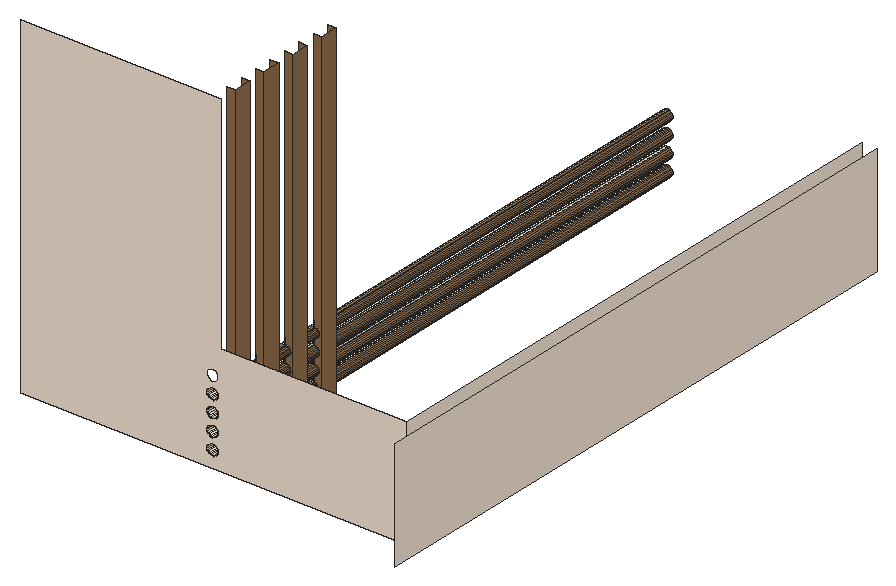
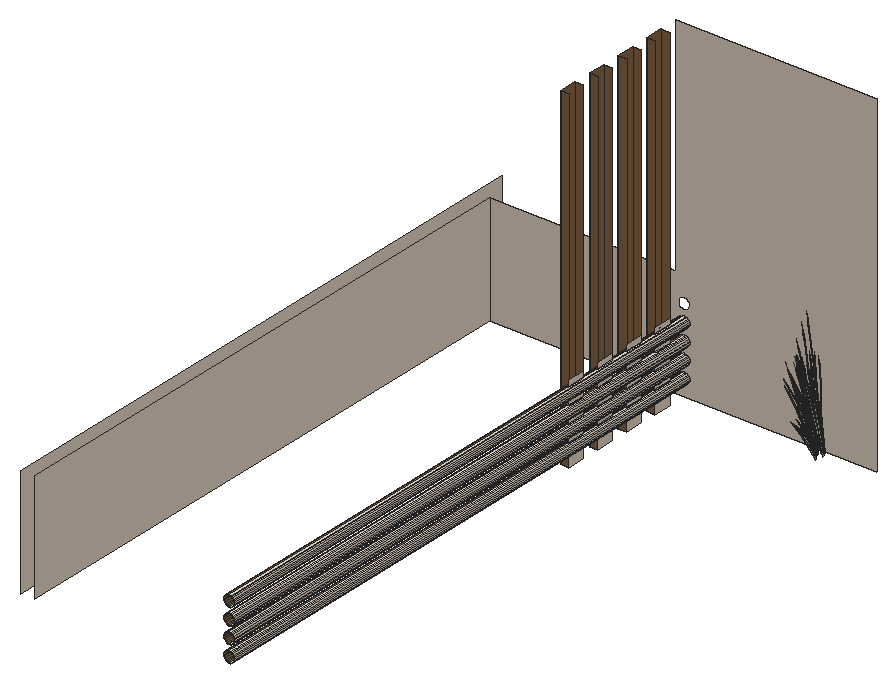
# SketchUp Ruby script. Lengths in inches.
U = 1.inch
M = Sketchup.active_model
def pt(a) = Geom::Point3d.new(a.map { |v| v * U })
def face(e, loops, mat)
  f = e.add_face(loops[0].map { |a| pt(a) })
  loops[1..].each { |l| e.add_face(l.map { |a| pt(a) }).erase! }
  f.material = f.back_material = mat if mat
  f
end
# faces: each face lists its corners as indices into pts; further lists are holes
def faces(e, pts, list, mat = nil) = list.each { |f| face(e, (f[0].is_a?(Array) ? f : [f]).map { |l| l.map { |i| pts[i] } }, mat) }
# xy, xz, yz: faces in a plane at the given z, y or x. An outline is a flat list of corners, or four numbers for a rectangle; further outlines are holes
def ring(l) = l.size == 4 ? [[l[0], l[1]], [l[2], l[1]], [l[2], l[3]], [l[0], l[3]]] : l.each_slice(2).to_a
def flat(e, list, mat, &to3) = list.each { |f| face(e, (f[0].is_a?(Array) ? f : [f]).map { |l| ring(l).map { |u, v| to3.(u, v) } }, mat) }
def xy(e, z, list, mat = nil) = flat(e, list, mat) { |x, y| [x, y, z] }
def xz(e, y, list, mat = nil) = flat(e, list, mat) { |x, z| [x, y, z] }
def yz(e, x, list, mat = nil) = flat(e, list, mat) { |y, z| [x, y, z] }
def lines(e, pts, list) = list.each { |a, b| e.add_line(pt(pts[a]), pt(pts[b])) }
# prism: a flat outline (further loops are holes) pulled along v
def prism(e, loops, v, mat = nil)
  f = face(e, loops, mat); d = Geom::Vector3d.new(v.map { |x| x * U })
  f.pushpull(f.normal.samedirection?(d) ? d.length : -d.length)
end
def box(e, o, s, mat = nil) = prism(e, [[o, [o[0] + s[0], o[1], o[2]], [o[0] + s[0], o[1] + s[1], o[2]], [o[0], o[1] + s[1], o[2]]]], [0, 0, s[2]], mat)
def at(x, y, z, deg = 0) = Geom::Transformation.translation(pt([x, y, z])) * Geom::Transformation.rotation(ORIGIN, Z_AXIS, deg.degrees)
def axes(o, x, y, z) = Geom::Transformation.new([*x, 0, *y, 0, *z, 0, *pt(o).to_a, 1])
def part(name) = M.definitions.add(name)
# library, detail: a bought-in or finely detailed component or shape, given as its bounding box
def library(name, o, s) = part(name).tap { |d| box(d.entities, o, s) }
def detail(e, o, s) = box(e.add_group.entities, o, s)
def put(e, d, t, mat = nil) = e.add_instance(d, t).tap { |i| i.material = mat if mat }
def group(e, t, mat = nil) = e.add_group.tap { |g| g.transformation = t; g.material = mat if mat }.entities
root = M.entities
M.materials.add("C01_Vanilla_Cream").color = [244, 228, 212]
M.materials.add("LightPink_Translucent").color = [144, 107, 117]
M.materials["LightPink_Translucent"].alpha = 0.75
M.materials.add("Wood_Floor_01_1K").color = [146, 111, 76]
c1 = part("blade")
p = [[2.15,0.21,22],[0,0.17,0],[0.09,0.45,0],[2.18,0.31,22],[2.29,0.31,22],[0.38,0.45,0],
  [2.48,0.24,33],[2.49,0.24,33],[2.48,0.22,33]]
faces(c1.entities,p,[[0,1,2,3],[4,5,2,3],[6,3,4,7],[8,0,3,6]])
c2 = part("seeds")
p = [[0.3,-0.1,1.38],[-0.01,-0.03,1.59],[-0.01,-0.03,0.03],[0.14,-0.07,-0.07],[0.29,-0.03,3],[0.15,0.01,3.11]]
faces(c2.entities,p,[[0,1,2,3],[1,0,4,5]],"LightPink_Translucent")
c3 = part("blade with seeds")
put(c3.entities,c1,at(0,0,0))
put(c3.entities,c2,axes([2.4,0.25,30.99],[1.5799,-0.05474,1.17369],[-0.12525,1.92788,0.29478],[-0.07173,-0.02425,1.56792]))
xy(root,12,[[357,18.46,360,24.91],[357,31.37,360,37.83],[357,44.28,360,50.74],[357,57.2,360,63.65]],"C01_Vanilla_Cream")
xz(root,12,[[[288,12,288,132,360,132,360,51.56,426.72,51.56,426.72,12],[357,16,357.52,16.07,358,16.27,358.41,16.59,358.73,17,358.93,17.48,359,18,358.93,18.52,358.73,19,358.41,19.41,358,19.73,357.52,19.93,357,20,356.48,19.93,356,19.73,355.59,19.41,355.27,19,355.07,18.52,355,18,355.07,17.48,355.27,17,355.59,16.59,356,16.27,356.48,16.07],[357,22,357.52,22.07,358,22.27,358.41,22.59,358.73,23,358.93,23.48,359,24,358.93,24.52,358.73,25,358.41,25.41,358,25.73,357.52,25.93,357,26,356.48,25.93,356,25.73,355.59,25.41,355.27,25,355.07,24.52,355,24,355.07,23.48,355.27,23,355.59,22.59,356,22.27,356.48,22.07],[357,28,357.52,28.07,358,28.27,358.41,28.59,358.73,29,358.93,29.48,359,30,358.93,30.52,358.73,31,358.41,31.41,358,31.73,357.52,31.93,357,32,356.48,31.93,356,31.73,355.59,31.41,355.27,31,355.07,30.52,355,30,355.07,29.48,355.27,29,355.59,28.59,356,28.27,356.48,28.07],[357,40,357.52,40.07,358,40.27,358.41,40.59,358.73,41,358.93,41.48,359,42,358.93,42.52,358.73,43,358.41,43.41,358,43.73,357.52,43.93,357,44,356.48,43.93,356,43.73,355.59,43.41,355.27,43,355.07,42.52,355,42,355.07,41.48,355.27,41,355.59,40.59,356,40.27,356.48,40.07],[357,34,357.52,34.07,358,34.27,358.41,34.59,358.73,35,358.93,35.48,359,36,358.93,36.52,358.73,37,358.41,37.41,358,37.73,357.52,37.93,357,38,356.48,37.93,356,37.73,355.59,37.41,355.27,37,355.07,36.52,355,36,355.07,35.48,355.27,35,355.59,34.59,356,34.27,356.48,34.07]]],"C01_Vanilla_Cream")
xz(root,18.46,[[357,12,360,132]],"Wood_Floor_01_1K")
xz(root,24.91,[[357,12,360,132]],"Wood_Floor_01_1K")
xz(root,31.37,[[357,12,360,132]],"Wood_Floor_01_1K")
xz(root,37.83,[[357,12,360,132]],"Wood_Floor_01_1K")
xz(root,44.28,[[357,12,360,132]],"Wood_Floor_01_1K")
xz(root,50.74,[[357,12,360,132]],"Wood_Floor_01_1K")
xz(root,57.2,[[357,12,360,132]],"Wood_Floor_01_1K")
xz(root,63.65,[[357,12,360,132]],"Wood_Floor_01_1K")
yz(root,357,[[18.46,12,24.91,16],[31.37,12,37.83,16],[44.28,12,50.74,16],[57.2,12,63.65,16],[18.46,16,24.91,20],
  [31.37,16,37.83,20],[44.28,16,50.74,20],[57.2,16,63.65,20],[18.46,20,24.91,22],[31.37,20,37.83,22],
  [44.28,20,50.74,22],[57.2,20,63.65,22],[18.46,22,24.91,26],[31.37,22,37.83,26],[44.28,22,50.74,26],
  [57.2,22,63.65,26],[18.46,26,24.91,28],[31.37,26,37.83,28],[44.28,26,50.74,28],[57.2,26,63.65,28],
  [18.46,28,24.91,32],[31.37,28,37.83,32],[44.28,28,50.74,32],[57.2,28,63.65,32],[18.46,32,24.91,34],
  [31.37,32,37.83,34],[44.28,32,50.74,34],[57.2,32,63.65,34],[18.46,34,24.91,38],[31.37,34,37.83,38],
  [44.28,34,50.74,38],[57.2,34,63.65,38],[18.46,38,24.91,40],[31.37,38,37.83,40],[44.28,38,50.74,40],
  [57.2,38,63.65,40]],"C01_Vanilla_Cream")
yz(root,360,[[18.46,12,24.91,132],[31.37,12,37.83,132],[44.28,12,50.74,132],[57.2,12,63.65,132]],"Wood_Floor_01_1K")
yz(root,426.72,[[12,12,216,51.56]],"C01_Vanilla_Cream")
yz(root,432,[[0,12,216,51.56]],"C01_Vanilla_Cream")
p = [[356.48,216,16.07],[357,216,16],[357,63.65,16],[357,57.2,16],[357,50.74,16],[357,44.28,16],
  [357,37.83,16],[357,31.37,16],[357,24.91,16],[357,18.46,16],[357,12,16],[356.48,12,16.07],
  [357.52,216,16.07],[357.52,12,16.07],[356,216,16.27],[356,12,16.27],[358,216,16.27],[358,12,16.27],
  [355.59,216,16.59],[355.59,12,16.59],[358.41,216,16.59],[358.41,12,16.59],[355.27,216,17],[355.27,12,17],
  [358.73,216,17],[358.73,12,17],[355.07,216,17.48],[355.07,12,17.48],[358.93,216,17.48],[358.93,12,17.48],
  [355,216,18],[355,12,18],[359,216,18],[359,12,18],[355.07,216,18.52],[355.07,12,18.52],
  [358.93,216,18.52],[358.93,12,18.52],[355.27,216,19],[355.27,12,19],[358.73,216,19],[358.73,12,19],
  [355.59,216,19.41],[355.59,12,19.41],[358.41,216,19.41],[358.41,12,19.41],[356,216,19.73],[356,12,19.73],
  [358,216,19.73],[358,12,19.73],[356.48,216,19.93],[356.48,12,19.93],[357.52,216,19.93],[357.52,12,19.93],
  [357,216,20],[357,12,20],[357,18.46,20],[357,24.91,20],[357,31.37,20],[357,37.83,20],
  [357,44.28,20],[357,50.74,20],[357,57.2,20],[357,63.65,20],[356.48,216,22.07],[357,216,22],
  [357,63.65,22],[357,57.2,22],[357,50.74,22],[357,44.28,22],[357,37.83,22],[357,31.37,22],
  [357,24.91,22],[357,18.46,22],[357,12,22],[356.48,12,22.07],[357.52,216,22.07],[357.52,12,22.07],
  [356,216,22.27],[356,12,22.27],[358,216,22.27],[358,12,22.27],[355.59,216,22.59],[355.59,12,22.59],
  [358.41,216,22.59],[358.41,12,22.59],[355.27,216,23],[355.27,12,23],[358.73,216,23],[358.73,12,23],
  [355.07,216,23.48],[355.07,12,23.48],[358.93,216,23.48],[358.93,12,23.48],[355,216,24],[355,12,24],
  [359,216,24],[359,12,24],[355.07,216,24.52],[355.07,12,24.52],[358.93,216,24.52],[358.93,12,24.52],
  [355.27,216,25],[355.27,12,25],[358.73,216,25],[358.73,12,25],[355.59,216,25.41],[355.59,12,25.41],
  [358.41,216,25.41],[358.41,12,25.41],[356,216,25.73],[356,12,25.73],[358,216,25.73],[358,12,25.73],
  [356.48,216,25.93],[356.48,12,25.93],[357.52,216,25.93],[357.52,12,25.93],[357,216,26],[357,12,26],
  [357,18.46,26],[357,24.91,26],[357,31.37,26],[357,37.83,26],[357,44.28,26],[357,50.74,26],
  [357,57.2,26],[357,63.65,26],[356.48,216,28.07],[357,216,28],[357,63.65,28],[357,57.2,28],
  [357,50.74,28],[357,44.28,28],[357,37.83,28],[357,31.37,28],[357,24.91,28],[357,18.46,28],
  [357,12,28],[356.48,12,28.07],[357.52,216,28.07],[357.52,12,28.07],[356,216,28.27],[356,12,28.27],
  [358,216,28.27],[358,12,28.27],[355.59,216,28.59],[355.59,12,28.59],[358.41,216,28.59],[358.41,12,28.59],
  [355.27,216,29],[355.27,12,29],[358.73,216,29],[358.73,12,29],[355.07,216,29.48],[355.07,12,29.48],
  [358.93,216,29.48],[358.93,12,29.48],[355,216,30],[355,12,30],[359,216,30],[359,12,30],
  [355.07,216,30.52],[355.07,12,30.52],[358.93,216,30.52],[358.93,12,30.52],[355.27,216,31],[355.27,12,31],
  [358.73,216,31],[358.73,12,31],[355.59,216,31.41],[355.59,12,31.41],[358.41,216,31.41],[358.41,12,31.41],
  [356,216,31.73],[356,12,31.73],[358,216,31.73],[358,12,31.73],[356.48,216,31.93],[356.48,12,31.93],
  [357.52,216,31.93],[357.52,12,31.93],[357,216,32],[357,12,32],[357,18.46,32],[357,24.91,32],
  [357,31.37,32],[357,37.83,32],[357,44.28,32],[357,50.74,32],[357,57.2,32],[357,63.65,32],
  [356.48,216,34.07],[357,216,34],[357,63.65,34],[357,57.2,34],[357,50.74,34],[357,44.28,34],
  [357,37.83,34],[357,31.37,34],[357,24.91,34],[357,18.46,34],[357,12,34],[356.48,12,34.07],
  [357.52,216,34.07],[357.52,12,34.07],[356,216,34.27],[356,12,34.27],[358,216,34.27],[358,12,34.27],
  [355.59,216,34.59],[355.59,12,34.59],[358.41,216,34.59],[358.41,12,34.59],[355.27,216,35],[355.27,12,35],
  [358.73,216,35],[358.73,12,35],[355.07,216,35.48],[355.07,12,35.48],[358.93,216,35.48],[358.93,12,35.48],
  [355,216,36],[355,12,36],[359,216,36],[359,12,36],[355.07,216,36.52],[355.07,12,36.52],
  [358.93,216,36.52],[358.93,12,36.52],[355.27,216,37],[355.27,12,37],[358.73,216,37],[358.73,12,37],
  [355.59,216,37.41],[355.59,12,37.41],[358.41,216,37.41],[358.41,12,37.41],[356,216,37.73],[356,12,37.73],
  [358,216,37.73],[358,12,37.73],[357,216,38],[356.48,216,37.93],[356.48,12,37.93],[357,12,38],
  [357,18.46,38],[357,24.91,38],[357,31.37,38],[357,37.83,38],[357,44.28,38],[357,50.74,38],
  [357,57.2,38],[357,63.65,38],[357.52,216,37.93],[357.52,12,37.93]]
faces(root,p,[[0,1,2,3,4,5,6,7,8,9,10,11],[14,0,11,15],[18,14,15,19],[22,18,19,23],[26,22,23,27],[30,26,27,31],[34,30,31,35],[38,34,35,39],
  [42,38,39,43],[46,42,43,47],[50,46,47,51],[54,50,51,55,56,57,58,59,60,61,62,63],[64,65,66,67,68,69,70,71,72,73,74,75],[78,64,75,79],[82,78,79,83],[86,82,83,87],
  [90,86,87,91],[94,90,91,95],[98,94,95,99],[102,98,99,103],[106,102,103,107],[110,106,107,111],[114,110,111,115],[118,114,115,119,120,121,122,123,124,125,126,127],
  [128,129,130,131,132,133,134,135,136,137,138,139],[142,128,139,143],[146,142,143,147],[150,146,147,151],[154,150,151,155],[158,154,155,159],[162,158,159,163],[166,162,163,167],
  [170,166,167,171],[174,170,171,175],[178,174,175,179],[182,178,179,183,184,185,186,187,188,189,190,191],[192,193,194,195,196,197,198,199,200,201,202,203],[206,192,203,207],[210,206,207,211],[214,210,211,215],
  [218,214,215,219],[222,218,219,223],[226,222,223,227],[230,226,227,231],[234,230,231,235],[238,234,235,239],[242,243,244,245,246,247,248,249,250,251,252,253]],"C01_Vanilla_Cream")
faces(root,p,[[1,12,13,10,9,8,7,6,5,4,3,2],[12,16,17,13],[16,20,21,17],[20,24,25,21],[24,28,29,25],[28,32,33,29],[32,36,37,33],[36,40,41,37],
  [40,44,45,41],[44,48,49,45],[48,52,53,49],[52,54,63,62,61,60,59,58,57,56,55,53],[65,76,77,74,73,72,71,70,69,68,67,66],[76,80,81,77],[80,84,85,81],[84,88,89,85],
  [88,92,93,89],[92,96,97,93],[96,100,101,97],[100,104,105,101],[104,108,109,105],[108,112,113,109],[112,116,117,113],[116,118,127,126,125,124,123,122,121,120,119,117],
  [129,140,141,138,137,136,135,134,133,132,131,130],[140,144,145,141],[144,148,149,145],[148,152,153,149],[152,156,157,153],[156,160,161,157],[160,164,165,161],[164,168,169,165],
  [168,172,173,169],[172,176,177,173],[176,180,181,177],[180,182,191,190,189,188,187,186,185,184,183,181],[193,204,205,202,201,200,199,198,197,196,195,194],[204,208,209,205],[208,212,213,209],[212,216,217,213],
  [216,220,221,217],[220,224,225,221],[224,228,229,225],[228,232,233,229],[232,236,237,233],[236,240,241,237],[254,242,253,252,251,250,249,248,247,246,245,255]],"Wood_Floor_01_1K")
put(root,c3,axes([298.97,21.29,18.38],[0.34808,-0.49367,0],[0.58235,0.27531,-0.38706],[0.13264,0.0627,1.22783]))
put(root,c3,axes([299.56,21.08,17.72],[-0.08333,-0.03881,1.32257],[-0.21404,-0.4336,-0.20205],[0.14439,-0.11767,0.22528]))
put(root,c3,axes([299.1,24.23,20.39],[-0.31678,-0.30846,0.2656],[0.36171,-0.29199,-0.3429],[0.18378,0.04443,0.65611]))
put(root,c3,axes([299.29,21.59,18.12],[0.52105,0.24633,-0.37238],[-0.31144,0.44171,0],[0.11867,0.0561,1.18128]))
put(root,c3,axes([299.39,24.51,20.15],[-0.02803,0.37463,0.04823],[-0.42332,-0.01027,0.37966],[0.16216,0.0392,0.57892]))
put(root,c3,axes([299.26,25.09,17.72],[0.04056,-0.07113,1.32257],[0.51066,-0.20948,-0.20205],[0.15482,0.10842,0.22528]))
put(root,c3,axes([299.42,24.39,20.15],[-0.41051,0.32462,0.36002],[-0.35404,-0.34474,0.29685],[0.1926,0.05988,0.74497]))
put(root,c3,axes([299.54,22.12,20.11],[-0.14302,-0.44985,-0.38324],[0.54163,-0.07869,-0.29685],[0.15522,-0.12083,0.7333]))
put(root,c3,axes([300.49,24.44,19.55],[-0.10656,-0.41414,-0.02619],[0.50364,-0.09521,-0.11874],[0.10517,0.02626,0.39164]))
put(root,c3,axes([299.62,23.37,20.39],[-0.46269,-0.13744,0.2656],[0.13495,-0.40096,-0.3429],[0.18628,-0.03677,0.65611]))
put(root,c3,axes([298.53,22.53,18.15],[0.57914,0.08077,-0.46765],[-0.12221,0.49823,-0.12274],[0.17283,0.06037,1.03225]))
put(root,c3,axes([301,22.83,18.3],[-0.34516,-0.31503,-0.04866],[0.37803,-0.28865,-0.22062],[0.10711,-0.02032,0.72768]))
put(root,c3,axes([300.2,21.22,18.68],[-0.18544,0.25079,0.86145],[-0.15939,-0.33694,0.63294],[0.15316,-0.08443,0.18974]))
put(root,c3,axes([299.98,22.34,20.15],[0.3822,0.20719,0.04823],[-0.22252,0.29505,0.37966],[0.12254,-0.09539,0.57892]))
put(root,c3,axes([299.875,22.25,20.15],[0.13808,0.45342,0.36002],[-0.54163,0.07869,0.29685],[0.15963,-0.10664,0.74497]))
put(root,c3,axes([298.41,23.6,19.51],[-0.2068,-0.08488,1.28532],[0.42797,-0.35609,0.10393],[0.26673,0.16064,0.54946]))
put(root,c3,axes([301.0625,22.32,20.13],[-0.07272,-0.00374,1.33037],[-0.30197,-0.40092,-0.12571],[0.12127,-0.13182,0.23543]))
put(root,c3,axes([299.9375,22.17,20],[0.48462,-0.07041,-0.2656],[0.12797,0.4025,0.3429],[0.13888,-0.10811,0.65611]))
put(root,c3,axes([299.55,22.3,20.34],[0.29081,-0.38873,-0.53284],[0.5096,0.27626,0.0643],[0.17364,-0.14084,0.75375]))
put(root,c3,axes([300.04,23.49,20.15],[0.20448,0.33592,0.04823],[-0.37288,0.16442,0.37966],[0.16437,-0.03244,0.57892]))
put(root,c3,axes([299.55,24.39,20],[0.31678,0.30846,-0.2656],[-0.36171,0.29199,0.3429],[0.18378,0.04443,0.65611]))
put(root,c3,axes([299.19,24.43,20.38],[0.02981,-0.50103,-0.0912],[0.56442,0.01369,-0.50621],[0.21738,0.0348,0.76918]))
put(root,c3,axes([299.81,23.5,20.38],[-0.28012,-0.44611,-0.0912],[0.49717,-0.21923,-0.50621],[0.20951,-0.05886,0.76918]))
put(root,c3,axes([300,23.37,20.15],[-0.15729,0.44921,0.36002],[-0.51712,-0.15361,0.29685],[0.20336,-0.027,0.74497]))
put(root,c3,axes([299.68,24.125,20.14],[0.11943,-0.00833,1.31208],[0.32759,-0.38275,-0.2075],[0.21244,0.05052,0.10523]))
put(root,c3,axes([299.79,23.12,20.11],[0.15083,-0.44814,-0.38324],[0.51712,0.15361,-0.29685],[0.2082,-0.04109,0.7333]))
put(root,c3,axes([301.09,23.4,18.68],[-0.34399,0.08133,0.86145],[0.16192,-0.33614,0.63294],[0.18249,0.023,0.18974]))
put(root,c3,axes([299.97,21.94,18.55],[-0.19889,-0.01459,1.07251],[-0.20376,-0.39145,-0.23066],[0.24434,-0.11074,0.45856]))
put(root,c3,axes([300.11,23.32,20],[0.46269,0.13744,-0.2656],[-0.13495,0.40096,0.3429],[0.18628,-0.03677,0.65611]))
put(root,c3,axes([299.21,24.1875,20.34],[0.55654,0.01186,-0.53284],[-0.03738,0.49951,0.0643],[0.23578,0.05271,0.75375]))
put(root,c3,axes([300.34,23.24,18.09],[-0.35858,0.05912,1.06187],[-0.05708,-0.47061,0.06078],[0.25115,-0.07123,0.60425]))
put(root,c3,axes([300.73,22.9375,17.72],[-0.0291,-0.0748,1.32257],[0.20181,-0.43752,-0.20205],[0.20357,-0.00629,0.22528]))
put(root,c3,axes([300.93,24.83,20.13],[-0.05034,-0.04313,1.33037],[0.11012,-0.46232,-0.12571],[0.1983,-0.02954,0.23543]))
put(root,c3,axes([298.85,22.83,19.51],[-0.23093,0.01116,1.28532],[0.15319,-0.4836,0.10393],[0.32909,0.02991,0.54946]))
put(root,c3,axes([299.69,23.28,20.34],[0.48922,-0.21758,-0.53284],[0.27264,0.44789,0.0643],[0.23638,-0.05088,0.75375]))
put(root,c3,axes([301.34,22.8,20.14],[0.07726,-0.07504,1.31208],[-0.09888,-0.46032,-0.2075],[0.19384,-0.08728,0.10523]))
put(root,c3,axes([300.44,23.94,18.55],[-0.13408,-0.12117,1.07251],[0.17446,-0.40083,-0.23066],[0.27128,0.0543,0.45856]))
